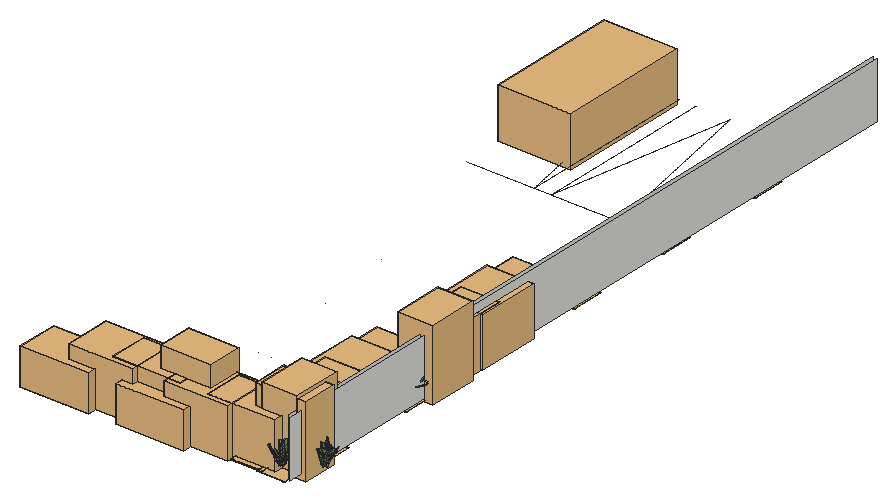
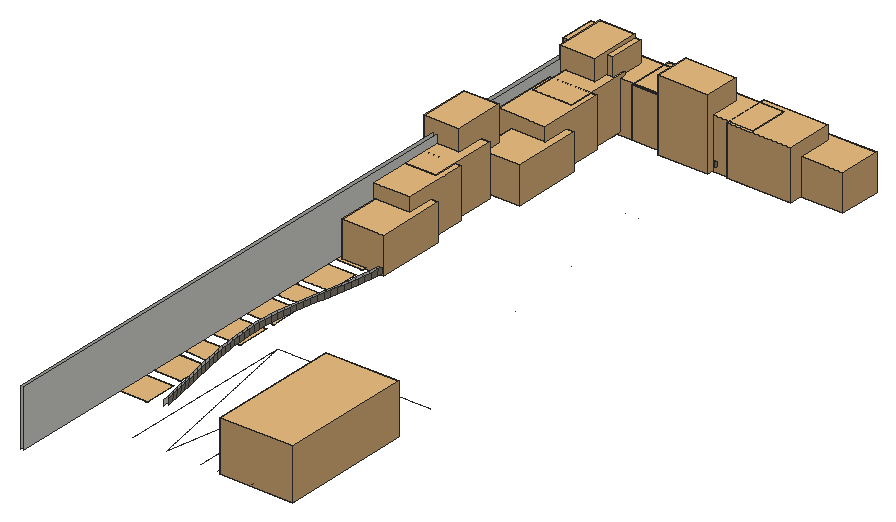
# SketchUp Ruby script. Lengths in inches.
U = 1.inch
M = Sketchup.active_model
def pt(a) = Geom::Point3d.new(a.map { |v| v * U })
def face(e, loops, mat)
  f = e.add_face(loops[0].map { |a| pt(a) })
  loops[1..].each { |l| e.add_face(l.map { |a| pt(a) }).erase! }
  f.material = f.back_material = mat if mat
  f
end
# faces: each face lists its corners as indices into pts; further lists are holes
def faces(e, pts, list, mat = nil) = list.each { |f| face(e, (f[0].is_a?(Array) ? f : [f]).map { |l| l.map { |i| pts[i] } }, mat) }
# xy, xz, yz: faces in a plane at the given z, y or x. An outline is a flat list of corners, or four numbers for a rectangle; further outlines are holes
def ring(l) = l.size == 4 ? [[l[0], l[1]], [l[2], l[1]], [l[2], l[3]], [l[0], l[3]]] : l.each_slice(2).to_a
def flat(e, list, mat, &to3) = list.each { |f| face(e, (f[0].is_a?(Array) ? f : [f]).map { |l| ring(l).map { |u, v| to3.(u, v) } }, mat) }
def xy(e, z, list, mat = nil) = flat(e, list, mat) { |x, y| [x, y, z] }
def xz(e, y, list, mat = nil) = flat(e, list, mat) { |x, z| [x, y, z] }
def yz(e, x, list, mat = nil) = flat(e, list, mat) { |y, z| [x, y, z] }
def lines(e, pts, list) = list.each { |a, b| e.add_line(pt(pts[a]), pt(pts[b])) }
# prism: a flat outline (further loops are holes) pulled along v
def prism(e, loops, v, mat = nil)
  f = face(e, loops, mat); d = Geom::Vector3d.new(v.map { |x| x * U })
  f.pushpull(f.normal.samedirection?(d) ? d.length : -d.length)
end
def box(e, o, s, mat = nil) = prism(e, [[o, [o[0] + s[0], o[1], o[2]], [o[0] + s[0], o[1] + s[1], o[2]], [o[0], o[1] + s[1], o[2]]]], [0, 0, s[2]], mat)
def at(x, y, z, deg = 0) = Geom::Transformation.translation(pt([x, y, z])) * Geom::Transformation.rotation(ORIGIN, Z_AXIS, deg.degrees)
def axes(o, x, y, z) = Geom::Transformation.new([*x, 0, *y, 0, *z, 0, *pt(o).to_a, 1])
def part(name) = M.definitions.add(name)
# library, detail: a bought-in or finely detailed component or shape, given as its bounding box
def library(name, o, s) = part(name).tap { |d| box(d.entities, o, s) }
def detail(e, o, s) = box(e.add_group.entities, o, s)
def put(e, d, t, mat = nil) = e.add_instance(d, t).tap { |i| i.material = mat if mat }
def group(e, t, mat = nil) = e.add_group.tap { |g| g.transformation = t; g.material = mat if mat }.entities
root = M.entities
M.materials.add("Material__4").color = [36, 36, 36]
M.materials.add("Material__6").color = [79, 108, 5]
M.materials.add("Plaster_06_1K").color = [141, 135, 122]
M.materials.add("calathea lutea").color = [121, 145, 80]
c1 = library("Group\#1",[4.11,-0.9,0],[77.07,140.59,53.39])
c2 = part("Group\#156")
g1 = group(c2.entities,at(8.61,38.85,0))
xy(g1,0,[[0,0,2.82,19.1,22.58,0],[22.58,0,2.82,19.1,22.58,19.1]],"calathea lutea")
p = [[2.82,19.1,0],[7.19,48.22,5.13],[10.77,48.22,5.13],[12.74,48.22,5.13],[22.58,48.22,5.13],[22.58,19.1,0]]
faces(g1,p,[[0,1,2,3,4,5]],"calathea lutea")
g2 = group(c2.entities,at(-0.77,-7.77,0))
p = [[14.8125,23.31,1.46],[21.35,23.31,0],[14.8125,0,1.46],[21.35,0,0],[27.89,0,1.46],[27.89,23.31,1.46],
  [8.27,46.62,2.92],[21.35,46.62,0],[34.4375,46.62,2.92],[4.47,23.31,6.43],[0,0,8.59],[33.76,0,4.28],
  [33.76,23.31,4.28]]
faces(g2,p,[[0,1,2],[3,2,1],[4,3,5],[1,5,3],[6,7,0],[1,0,7],[5,1,8],[7,8,1],
  [9,0,2,10],[11,4,5,12],[9,6,0],[12,5,8]],"calathea lutea")
c3 = part("Group\#150")
xy(c3.entities,0,[[0,0,0,33.87,27.21,33.87,19.71,0]],"calathea lutea")
c4 = part("Group\#157")
xy(c4.entities,1.04,[[21.13,33.87,21.13,57.59,32.375,57.59,27.12,33.87]],"calathea lutea")
xy(c4.entities,1.32,[[0.12,33.87,7.74,57.59]],"calathea lutea")
p = [[7.74,33.87,1.32],[11.8,57.59,0.61],[15.24,57.59,0],[15.24,33.87,0],[18.43,57.59,0.5625],[21.13,57.59,1.04],
  [21.13,33.87,1.04],[15.24,77.7,2.36],[21.13,77.7,3.4],[7.74,57.59,1.32],[7.74,77.7,3.69],[36.83,77.7,3.4],
  [32.375,57.59,1.04],[0.12,57.59,1.32],[0.12,77.7,3.69]]
faces(c4.entities,p,[[0,1,2,3],[3,2,4],[3,4,5,6],[7,2,1],[8,4,2,7],[0,9,1],[7,1,9,10],[8,5,4],
  [11,12,5,8],[10,9,13,14]],"calathea lutea")
put(c4.entities,c3,axes([0,-16.9375,0],[1,0,0],[0,1.5,0],[0,0,1]))
c5 = part("Group\#155")
g3 = group(c5.entities,at(0,-17.3,0))
xy(g3,0,[[0,0,28.07,51.9]],"calathea lutea")
g4 = group(c5.entities,at(0.9,34.6,0))
xy(g4,0,[[13.14,0,13.14,26.22,16.85,26.22],[13.14,0,16.85,26.22,20.16,26.22,20.16,0]],"calathea lutea")
p = [[6.36,0,1.82],[9.95,26.22,0.86],[13.14,26.22,0],[13.14,0,0],[20.16,0,0],[20.16,26.22,0],
  [27.07,26.22,1.22],[27.07,0,1.22],[13.14,49.5625,5.91],[20.16,49.5625,5.91],[16.85,26.22,0],[27.07,49.5625,7.125],
  [6.36,26.22,1.82],[6.36,49.5625,7.72],[0,0,4.78],[0,26.22,4.78],[0,49.5625,10.6875]]
faces(g4,p,[[0,1,2,3],[4,5,6,7],[8,2,1],[9,10,2,8],[9,5,10],[11,6,5,9],[0,12,1],[8,1,12,13],
  [14,15,12,0],[13,12,15,16]],"calathea lutea")
c6 = part("Group\#154")
put(c6.entities,c3,axes([0,-16.9375,0],[1,0,0],[0,1.5,0],[0,0,1]))
g5 = group(c6.entities,at(-0.23,33.4,-0.35))
p = [[15.12,39.14,-19.87],[15.12,20.54,-11.86],[11.68,20.84,-11.33],[21.02,39.66,-18.97],[18.3125,20.82,-11.37],[7.62,21.2,-10.71],
  [7.62,39.8,-18.72],[21.02,21.06,-10.96],[36.72,39.66,-18.97],[32.26,21.06,-10.96],[0,21.2,-10.71],[0,39.8,-18.72],
  [7.62,0.66,1.15],[15.12,0,0],[21.02,0.52,0.9],[27.01,0.52,0.9],[0,0.66,1.15]]
faces(g5,p,[[0,1,2],[3,4,1,0],[0,2,5,6],[3,7,4],[8,9,7,3],[6,5,10,11],[12,2,1,13],[13,1,4],
  [13,4,7,14],[12,5,2],[14,7,9,15],[16,10,5,12]],"calathea lutea")
c7 = part("Foliage cluster")
put(c7.entities,c2,axes([37.24,8.07,75.17],[1,0,0],[0,0.45554,-0.89021],[0,0.89021,0.45554]))
put(c7.entities,c4,axes([69.44,65.48,16.68],[-0.53288,-0.84619,0],[0.14694,-0.09253,0.98481],[-0.83334,0.52478,0.17365]))
put(c7.entities,c5,axes([47.9375,70.43,17.04],[0.74664,-0.66523,0],[0.11552,0.12965,0.98481],[-0.65512,-0.7353,0.17365]))
put(c7.entities,c2,axes([76.19,10.66,75.17],[0.70711,0.70711,0],[-0.32212,0.32212,-0.89021],[-0.62948,0.62948,0.45554]))
put(c7.entities,c2,axes([101.91,40.03,75.17],[0,1,0],[-0.45554,0,-0.89021],[-0.89021,0,0.45554]))
put(c7.entities,c2,axes([99.32,78.99,75.17],[-0.70711,0.70711,0],[-0.32212,-0.32212,-0.89021],[-0.62948,-0.62948,0.45554]))
put(c7.entities,c5,axes([34.81,63.36,17.04],[0.99956,-0.02967,0],[0.00515,0.17357,0.98481],[-0.02922,-0.98437,0.17365]))
put(c7.entities,c5,axes([48,37.4,15.8],[-0.14436,0.98953,0],[-0.40248,-0.05871,0.91355],[0.90398,0.13188,0.40674]))
put(c7.entities,c4,axes([56.87,39.77,12.28],[-0.67695,0.4263,0],[-0.18016,-0.28609,0.72505],[0.38636,0.61353,0.33809]))
put(c7.entities,c4,axes([36.12,43.25,12.28],[0.18947,0.77724,0],[-0.32848,0.08007,0.72505],[0.70442,-0.17172,0.33809]))
put(c7.entities,c6,axes([35.1,54.93,11.375],[0.79719,0.06694,0],[-0.03636,0.43302,0.6717],[0.05621,-0.66934,0.43454]))
put(c7.entities,c4,axes([41.66,47.32,12.28],[0.45082,0.66088,0],[-0.2793,0.19053,0.72505],[0.59896,-0.40858,0.33809]))
put(c7.entities,c4,axes([47.89,59.4,12.28],[0.79719,0.06694,0],[-0.02829,0.33691,0.72505],[0.06067,-0.7225,0.33809]))
put(c7.entities,c6,axes([29.53,49.96,11.375],[0.65692,0.45657,0],[-0.248,0.35682,0.6717],[0.38335,-0.55156,0.43454]))
put(c7.entities,c6,axes([29.9,49.27,12.86],[0.34062,0.72386,0],[-0.22849,0.10752,0.7591],[0.68685,-0.32321,0.25252]))
put(c7.entities,c6,axes([36.33,48.82,8.99],[0.09232,0.62522,0],[-0.3396,0.05015,0.53064],[0.52495,-0.07752,0.34329]))
put(c7.entities,c6,axes([49.82,38.52,8.99],[-0.54622,0.31791,0],[-0.17268,-0.29669,0.53064],[0.26692,0.45862,0.34329]))
put(c7.entities,c6,axes([55.68,39.21,8.99],[-0.632,0.00221,0],[-0.0012,-0.34328,0.53064],[0.00185,0.53064,0.34329]))
c8 = library("Group\#28",[0,0,0],[86.94,78.77,46.4375])
c9 = library("Group\#14",[-978.71,-103.24,719.12],[90.2,76.4,68.29])
c10 = library("Group\#13",[-906.16,-138.28,686.8],[98.25,106.18,75.79])
c11 = library("Group\#202",[-3.47,-2.45,12.47],[53.14,54.93,75.51])
c12 = part("Group\#44")
put(c12.entities,c7,axes([161.54,105.34,6.01],[0.19523,-0.19694,0],[0.19694,0.19523,0],[0,0,0.24957]))
put(c12.entities,c8,axes([0,37.34,0.92],[0.83,0,0],[0,0.83,0],[0,0,0.83]))
put(c12.entities,c9,axes([859.63,139.86,-568.1],[0.79,0,0],[0,0.79,0],[0,0,0.79]),"Material__4")
put(c12.entities,c10,axes([669.69,145.1,-472.48],[0.69,0,0],[0,0.69,0],[0,0,0.69]),"Material__6")
put(c12.entities,c11,at(132.78,74.93,-12.6))
c13 = library("t1",[-17.79,-17.21,0],[35.58,34.42,0.01])
c14 = library("tt",[-12.4,-12.1,0],[24.8,24.2,0.01])
c15 = library("ew",[-14.92,-16.84,0],[29.84,33.68,0.01])
yz(root,1204.463,[[4.952,0,777.168,60]])
yz(root,1208.463,[[0.952,0,777.168,60]])
p = [[1173.842,30.55,0],[1184.195,25.466,0],[1184.195,25.466,6],[1173.842,30.55,6],[1183.794,26.3125,0],[1183.794,26.3125,6],
  [1183.284,27.387,0],[1183.284,27.387,6],[1182.372,29.308,0],[1182.372,29.308,6],[1181.461,31.229,0],[1181.461,31.229,6],
  [1163.128,34.769,0],[1163.128,34.769,6],[1180.549,33.15,0],[1180.549,33.15,6],[1177.627,32.131,0],[1166.497,36.747,0],
  [1166.497,36.747,6],[1177.627,32.131,6],[1176.661,34.304,0],[1176.661,34.304,6],[1179.638,35.072,0],[1179.638,35.072,6],
  [1175.695,36.527,0],[1175.695,36.527,6],[1152.093,38.186,0],[1152.093,38.186,6],[1178.718,37.074,0],[1178.718,37.074,6],
  [1174.719,39.093,0],[1174.719,39.093,6],[1155.033,40.481,0],[1155.033,40.481,6],[1177.76,39.506,0],[1177.76,39.506,6],
  [1140.779,40.863,0],[1140.779,40.863,6],[1173.734,42.055,0],[1173.734,42.055,6],[1010.869,39.548,0],[1022.293,40.839,0],
  [1022.293,40.839,6],[1010.869,39.548,6],[1176.771,42.402,0],[1176.771,42.402,6],[1143.285,43.404,0],[1143.285,43.404,6],
  [1033.892,42.071,0],[1033.892,42.071,6],[1129.231,42.863,0],[1129.231,42.863,6],[1045.666,43.202,0],[1045.666,43.202,6],
  [1172.739,45.418,0],[1172.739,45.418,6],[1175.76,45.758,0],[1175.76,45.758,6],[1117.493,44.247,0],[1117.493,44.247,6],
  [1057.573,44.168,0],[1057.573,44.168,6],[1131.302,45.588,0],[1131.302,45.588,6],[1032.854,44.981,0],[1020.952,43.709,0],
  [1020.952,43.709,6],[1032.854,44.981,6],[1069.567,44.904,0],[1069.567,44.904,6],[1105.612,45.08,0],[1105.612,45.08,6],
  [1081.602,45.344,0],[1081.602,45.344,6],[1044.954,46.15,0],[1044.954,46.15,6],[1093.632,45.424,0],[1093.632,45.424,6],
  [1171.734,49.186,0],[1171.734,49.186,6],[1119.133,47.104,0],[1119.133,47.104,6],[1174.731,49.573,0],[1174.731,49.573,6],
  [1057.211,47.15,0],[1057.211,47.15,6],[1069.575,47.908,0],[1069.575,47.908,6],[1106.827,48.023,0],[1106.827,48.023,6],
  [1081.999,48.353,0],[1081.999,48.353,6],[1094.433,48.415,0],[1094.433,48.415,6],[1170.719,53.365,0],[1170.719,53.365,6],
  [1173.687,53.849,0],[1173.687,53.849,6],[1169.695,57.96,0],[1169.695,57.96,6],[1172.628,58.59,0],[1172.628,58.59,6],
  [1168.661,62.975,0],[1168.661,62.975,6],[1171.556,63.797,0],[1171.556,63.797,6],[1167.617,68.415,0],[1167.617,68.415,6],
  [1170.472,69.476,0],[1170.472,69.476,6],[1166.557,74.284,0],[1166.557,74.284,6],[1169.362,75.643,0],[1169.362,75.643,6],
  [1165.459,80.555,0],[1165.459,80.555,6],[1168.217,82.236,0],[1168.217,82.236,6],[1164.367,87.17,0],[1164.367,87.17,6],
  [1167.089,89.177,0],[1167.089,89.177,6],[1163.328,94.072,0],[1163.328,94.072,6],[1166.033,96.404,0],[1166.033,96.404,6],
  [1162.393,101.204,0],[1162.393,101.204,6],[1165.106,103.848,0],[1165.106,103.848,6],[1161.61,108.508,0],[1161.61,108.508,6],
  [1164.362,111.445,0],[1164.362,111.445,6],[1161.028,115.926,0],[1161.028,115.926,6],[1163.855,119.127,0],[1163.855,119.127,6],
  [1160.696,123.401,0],[1160.696,123.401,6],[1163.641,126.824,0],[1163.641,126.824,6],[1160.663,130.876,0],[1160.663,130.876,6],
  [1163.772,134.471,0],[1163.772,134.471,6],[1160.979,138.293,0],[1160.979,138.293,6],[1164.302,141.997,0],[1164.302,141.997,6],
  [1161.693,145.594,0],[1161.693,145.594,6],[1165.28,149.333,0],[1165.28,149.333,6],[1162.854,152.722,0],[1162.854,152.722,6],
  [1166.75,156.442,0],[1166.75,156.442,6],[1164.468,159.642,0],[1164.468,159.642,6],[1168.646,163.4,0],[1168.646,163.4,6],
  [1166.419,166.384,0],[1166.419,166.384,6],[1170.819,170.259,0],[1170.819,170.259,6],[1168.568,172.991,0],[1168.568,172.991,6],
  [1173.117,177.07,0],[1173.117,177.07,6],[1170.775,179.506,0],[1170.775,179.506,6],[1175.383,183.882,0],[1175.383,183.882,6],
  [1172.9,185.972,0],[1172.9,185.972,6],[1177.455,190.748,0],[1177.455,190.748,6],[1174.806,192.43,0],[1174.806,192.43,6],
  [1179.166,197.72,0],[1179.166,197.72,6],[1176.351,198.924,0],[1176.351,198.924,6],[1180.346,204.83,0],[1180.346,204.83,6],
  [1177.405,205.495,0],[1177.405,205.495,6],[1180.942,212.025,0],[1180.942,212.025,6],[1177.944,212.156,0],[1177.944,212.156,6],
  [1181.012,219.283,0],[1181.012,219.283,6],[1178.02,218.902,0],[1178.02,218.902,6],[1177.683,225.73,0],[1177.683,225.73,6],
  [1180.624,226.599,0],[1180.624,226.599,6],[1176.987,232.633,0],[1176.987,232.633,6],[1179.842,233.968,0],[1179.842,233.968,6],
  [1175.982,239.607,0],[1175.982,239.607,6],[1178.729,241.385,0],[1178.729,241.385,6],[1174.722,246.647,0],[1174.722,246.647,6],
  [1177.347,248.847,0],[1177.347,248.847,6],[1173.258,253.748,0],[1173.258,253.748,6],[1175.758,256.349,0],[1175.758,256.349,6],
  [1171.641,260.906,0],[1171.641,260.906,6],[1174.022,263.888,0],[1174.022,263.888,6],[1169.925,268.115,0],[1169.925,268.115,6],
  [1172.201,271.46,0],[1172.201,271.46,6],[1168.162,275.37,0],[1168.162,275.37,6],[1170.354,279.059,0],[1170.354,279.059,6],
  [1166.402,282.667,0],[1166.402,282.667,6],[1168.539,286.68,0],[1168.539,286.68,6],[1164.699,290,0],[1164.699,290,6],
  [1166.816,294.318,0],[1166.816,294.318,6],[1163.104,297.365,0],[1163.104,297.365,6],[1165.243,301.966,0],[1165.243,301.966,6],
  [1161.669,304.757,0],[1161.669,304.757,6],[1163.879,309.619,0],[1163.879,309.619,6],[1160.447,312.17,0],[1160.447,312.17,6],
  [1162.781,317.269,0],[1162.781,317.269,6],[1159.489,319.601,0],[1159.489,319.601,6],[1162.005,324.913,0],[1162.005,324.913,6],
  [1158.845,327.044,0],[1158.845,327.044,6],[1161.575,332.569,0],[1161.575,332.569,6],[1158.519,334.496,0],[1158.519,334.496,6],
  [1161.469,340.244,0],[1161.469,340.244,6],[1158.486,341.954,0],[1158.486,341.954,6],[1161.656,347.937,0],[1161.656,347.937,6],
  [1158.72,349.418,0],[1158.72,349.418,6],[1162.11,355.645,0],[1162.11,355.645,6],[1159.197,356.884,0],[1159.197,356.884,6],
  [1162.803,363.366,0],[1162.803,363.366,6],[1159.889,364.351,0],[1159.889,364.351,6],[1163.705,371.097,0],[1163.705,371.097,6],
  [1160.772,371.816,0],[1160.772,371.816,6],[1164.788,378.836,0],[1164.788,378.836,6],[1161.82,379.278,0],[1161.82,379.278,6],
  [1166.023,386.58,0],[1166.023,386.58,6],[1163.007,386.735,0],[1163.007,386.735,6],[1167.382,394.326,0],[1167.382,394.326,6],
  [1164.306,394.184,0],[1164.306,394.184,6],[1165.693,401.623,0],[1165.693,401.623,6],[1168.835,402.073,0],[1168.835,402.073,6],
  [1167.142,409.051,0],[1167.142,409.051,6],[1170.353,409.818,0],[1170.353,409.818,6],[1168.627,416.465,0],[1168.627,416.465,6],
  [1171.908,417.557,0],[1171.908,417.557,6],[1170.122,423.863,0],[1170.122,423.863,6],[1173.47,425.29,0],[1173.47,425.29,6],
  [1171.601,431.244,0],[1171.601,431.244,6],[1175.009,433.013,0],[1175.009,433.013,6],[1173.039,438.604,0],[1173.039,438.604,6],
  [1176.496,440.724,0],[1176.496,440.724,6],[1174.41,445.943,0],[1174.41,445.943,6],[1177.901,448.421,0],[1177.901,448.421,6],
  [1175.689,453.258,0],[1175.689,453.258,6],[1179.195,456.103,0],[1179.195,456.103,6],[1176.848,460.546,0],[1176.848,460.546,6],
  [1180.347,463.768,0],[1180.347,463.768,6],[1177.864,467.806,0],[1177.864,467.806,6],[1181.329,471.412,0],[1181.329,471.412,6],
  [1178.71,475.037,0],[1178.71,475.037,6],[1182.108,479.036,0],[1182.108,479.036,6],[1179.36,482.234,0],[1179.36,482.234,6],
  [1182.656,486.633,0],[1182.656,486.633,6],[1179.793,489.398,0],[1179.793,489.398,6],[1182.963,494.191,0],[1182.963,494.191,6],
  [1180.012,496.53,0],[1180.012,496.53,6],[1183.044,501.71,0],[1183.044,501.71,6],[1180.03,503.631,0],[1180.03,503.631,6],
  [1182.914,509.189,0],[1182.914,509.189,6],[1179.862,510.703,0],[1179.862,510.703,6],[1182.589,516.632,0],[1182.589,516.632,6],
  [1179.519,517.75,0],[1179.519,517.75,6],[1182.084,524.038,0],[1182.084,524.038,6],[1179.016,524.773,0],[1179.016,524.773,6],
  [1181.414,531.411,0],[1181.414,531.411,6],[1178.365,531.775,0],[1178.365,531.775,6],[1180.596,538.751,0],[1180.596,538.751,6],
  [1177.58,538.758,0],[1177.58,538.758,6],[1176.674,545.723,0],[1176.674,545.723,6],[1179.645,546.06,0],[1179.645,546.06,6],
  [1175.661,552.674,0],[1175.661,552.674,6],[1178.576,553.341,0],[1178.576,553.341,6],[1174.552,559.613,0],[1174.552,559.613,6],
  [1177.405,560.595,0],[1177.405,560.595,6],[1173.363,566.542,0],[1173.363,566.542,6],[1176.148,567.823,0],[1176.148,567.823,6],
  [1172.106,573.462,0],[1172.106,573.462,6],[1174.819,575.029,0],[1174.819,575.029,6],[1170.794,580.377,0],[1170.794,580.377,6],
  [1173.433,582.212,0],[1173.433,582.212,6],[1169.441,587.289,0],[1169.441,587.289,6],[1172.007,589.376,0],[1172.007,589.376,6],
  [1168.059,594.2,0],[1168.059,594.2,6],[1170.555,596.522,0],[1170.555,596.522,6],[1166.663,601.112,0],[1166.663,601.112,6],
  [1169.092,603.651,0],[1169.092,603.651,6],[1165.264,608.027,0],[1165.264,608.027,6],[1167.634,610.766,0],[1167.634,610.766,6],
  [1163.878,614.947,0],[1163.878,614.947,6],[1166.195,617.869,0],[1166.195,617.869,6],[1162.516,621.876,0],[1162.516,621.876,6],
  [1164.792,624.96,0],[1164.792,624.96,6],[1161.192,628.815,0],[1161.192,628.815,6],[1163.439,632.043,0],[1163.439,632.043,6],
  [1159.92,635.766,0],[1159.92,635.766,6],[1162.151,639.118,0],[1162.151,639.118,6],[1158.712,642.732,0],[1158.712,642.732,6],
  [1160.942,646.187,0],[1160.942,646.187,6],[1044.376,252.565,0],[1044.376,252.562,0],[1075.57,512.779,0],[1075.57,704.823,0],
  [1075.568,512.78,0],[1111.697,704.824,0],[1183.8125,26.294,0],[1033.624,340.952,0],[1033.625,340.953,0],[1052.548,154.932,0],
  [1052.548,154.93,0],[1066.097,154.932,0],[1066.097,154.93,0],[985.675,512.779,0],[1057.718,512.779,0],[1057.718,704.823,0],
  [1021.589,704.824,0],[1147.611,512.78,0],[1147.612,512.779,0],[1147.612,704.823,0]]
faces(root,p,[[0,1,2,3],[1,4,5,2],[4,6,7,5],[6,8,9,7],[8,10,11,9],[12,0,3,13],[10,14,15,11],[14,22,23,15],
  [26,12,13,27],[22,28,29,23],[28,34,35,29],[36,26,27,37],[40,41,42,43],[34,44,45,35],[41,48,49,42],[50,36,37,51],
  [48,52,53,49],[44,56,57,45],[58,50,51,59],[52,60,61,53],[60,68,69,61],[70,58,59,71],[68,72,73,69],[76,70,71,77],
  [72,76,77,73],[56,82,83,57],[82,96,97,83],[96,100,101,97],[100,104,105,101],[104,108,109,105],[108,112,113,109],[112,116,117,113],
  [116,120,121,117],[120,124,125,121],[124,128,129,125],[128,132,133,129],[132,136,137,133],[136,140,141,137],[140,144,145,141],[144,148,149,145],
  [148,152,153,149],[152,156,157,153],[156,160,161,157],[160,164,165,161],[164,168,169,165],[168,172,173,169],[172,176,177,173],[176,180,181,177],
  [180,184,185,181],[184,188,189,185],[188,192,193,189],[192,198,199,193],[198,202,203,199],[202,206,207,203],[206,210,211,207],[210,214,215,211],
  [214,218,219,215],[218,222,223,219],[222,226,227,223],[226,230,231,227],[230,234,235,231],[234,238,239,235],[238,242,243,239],[242,246,247,243],
  [246,250,251,247],[250,254,255,251],[254,258,259,255],[258,262,263,259],[262,266,267,263],[266,270,271,267],[270,274,275,271],[274,278,279,275],
  [278,282,283,279],[282,286,287,283],[286,292,293,287],[292,296,297,293],[296,300,301,297],[300,304,305,301],[304,308,309,305],[308,312,313,309],
  [312,316,317,313],[316,320,321,317],[320,324,325,321],[324,328,329,325],[328,332,333,329],[332,336,337,333],[336,340,341,337],[340,344,345,341],
  [344,348,349,345],[348,352,353,349],[352,356,357,353],[356,360,361,357],[360,364,365,361],[364,370,371,365],[370,374,375,371],[374,378,379,375],
  [378,382,383,379],[382,386,387,383],[386,390,391,387],[390,394,395,391],[394,398,399,395],[398,402,403,399],[402,406,407,403],[406,410,411,407],
  [410,414,415,411],[414,418,419,415],[418,422,423,419],[422,426,427,423]])
faces(root,p,[[16,17,18,19],[20,16,19,21],[24,20,21,25],[30,24,25,31],[17,32,33,18],[38,30,31,39],[32,46,47,33],[54,38,39,55],
  [46,62,63,47],[64,65,66,67],[74,64,67,75],[78,54,55,79],[62,80,81,63],[84,74,75,85],[86,84,85,87],[80,88,89,81],
  [90,86,87,91],[88,92,93,89],[92,90,91,93],[94,78,79,95],[98,94,95,99],[102,98,99,103],[106,102,103,107],[110,106,107,111],
  [114,110,111,115],[118,114,115,119],[122,118,119,123],[126,122,123,127],[130,126,127,131],[134,130,131,135],[138,134,135,139],[142,138,139,143],
  [146,142,143,147],[150,146,147,151],[154,150,151,155],[158,154,155,159],[162,158,159,163],[166,162,163,167],[170,166,167,171],[174,170,171,175],
  [178,174,175,179],[182,178,179,183],[186,182,183,187],[190,186,187,191],[194,190,191,195],[196,194,195,197],[200,196,197,201],[204,200,201,205],
  [208,204,205,209],[212,208,209,213],[216,212,213,217],[220,216,217,221],[224,220,221,225],[228,224,225,229],[232,228,229,233],[236,232,233,237],
  [240,236,237,241],[244,240,241,245],[248,244,245,249],[252,248,249,253],[256,252,253,257],[260,256,257,261],[264,260,261,265],[268,264,265,269],
  [272,268,269,273],[276,272,273,277],[280,276,277,281],[284,280,281,285],[288,284,285,289],[290,288,289,291],[294,290,291,295],[298,294,295,299],
  [302,298,299,303],[306,302,303,307],[310,306,307,311],[314,310,311,315],[318,314,315,319],[322,318,319,323],[326,322,323,327],[330,326,327,331],
  [334,330,331,335],[338,334,335,339],[342,338,339,343],[346,342,343,347],[350,346,347,351],[354,350,351,355],[358,354,355,359],[362,358,359,363],
  [366,362,363,367],[368,366,367,369],[372,368,369,373],[376,372,373,377],[380,376,377,381],[384,380,381,385],[388,384,385,389],[392,388,389,393],
  [396,392,393,397],[400,396,397,401],[404,400,401,405],[408,404,405,409],[412,408,409,413],[416,412,413,417],[420,416,417,421],[424,420,421,425]],"Plaster_06_1K")
lines(root,p,[[428,429],[430,431],[432,433],[4,434],[435,436],[432,430],[437,438],[439,440],[441,442],[442,432],[443,442],[444,442],
  [430,445],[445,446],[433,445],[447,446]])
put(root,c1,axes([976.41,701.02,-3.87],[1,0,0],[0,-1,0],[0,0,1]))
put(root,c12,axes([930.34,-33.03,-5.25],[1,0,0],[0,0.67442,0],[0,0,1]))
put(root,c13,axes([1055.84,17.9375,0],[0,-1,0],[-1,0,0],[0,0,1]))
put(root,c14,axes([1083.21,18.42,0],[0,-1,0],[-1,0,0],[0,0,1]))
put(root,c15,axes([1119.65,20.08,0],[0,-1,0],[-1,0,0],[0,0,1]))
put(root,c12,axes([1031.13,-33.03,-5.25],[1,0,0],[0,0.67442,0],[0,0,1]))
put(root,c13,axes([1163.89,17.9375,0],[0,-1,0],[-1,0,0],[0,0,1]))
put(root,c12,axes([1118.65,197.49,-2.26],[0,-1,0],[0.67442,0,0],[0,0,1]))
put(root,c12,axes([1132.22,360.22,-2.26],[0,-1,0],[0.67442,0,0],[0,0,1]))
put(root,c15,axes([1191.02,14.09,0],[1,0,0],[0,-1,0],[0,0,1]))
put(root,c15,axes([1191.02,125.32,0],[1,0,0],[0,-1,0],[0,0,1]))
put(root,c15,axes([1191.02,227.12,0],[1,0,0],[0,-1,0],[0,0,1]))
put(root,c15,axes([1191.02,347.67,0],[1,0,0],[0,-1,0],[0,0,1]))
put(root,c15,axes([1191.02,465.72,0],[1,0,0],[0,-1,0],[0,0,1]))
put(root,c15,axes([1191.02,588.05,0],[1,0,0],[0,-1,0],[0,0,1]))
put(root,c14,axes([1192.68,88.88,0],[1,0,0],[0,-1,0],[0,0,1]))
put(root,c14,axes([1192.68,190.68,0],[1,0,0],[0,-1,0],[0,0,1]))
put(root,c14,axes([1192.68,311.23,0],[1,0,0],[0,-1,0],[0,0,1]))
put(root,c14,axes([1192.68,429.28,0],[1,0,0],[0,-1,0],[0,0,1]))
put(root,c14,axes([1192.68,551.62,0],[1,0,0],[0,-1,0],[0,0,1]))
put(root,c13,axes([1193.17,58.33,0],[1,0,0],[0,-1,0],[0,0,1]))
put(root,c13,axes([1193.17,169.56,0],[1,0,0],[0,-1,0],[0,0,1]))
put(root,c13,axes([1193.17,271.36,0],[1,0,0],[0,-1,0],[0,0,1]))
put(root,c13,axes([1193.17,391.91,0],[1,0,0],[0,-1,0],[0,0,1]))
put(root,c13,axes([1193.17,509.96,0],[1,0,0],[0,-1,0],[0,0,1]))
put(root,c13,axes([1193.17,632.29,0],[1,0,0],[0,-1,0],[0,0,1]))
